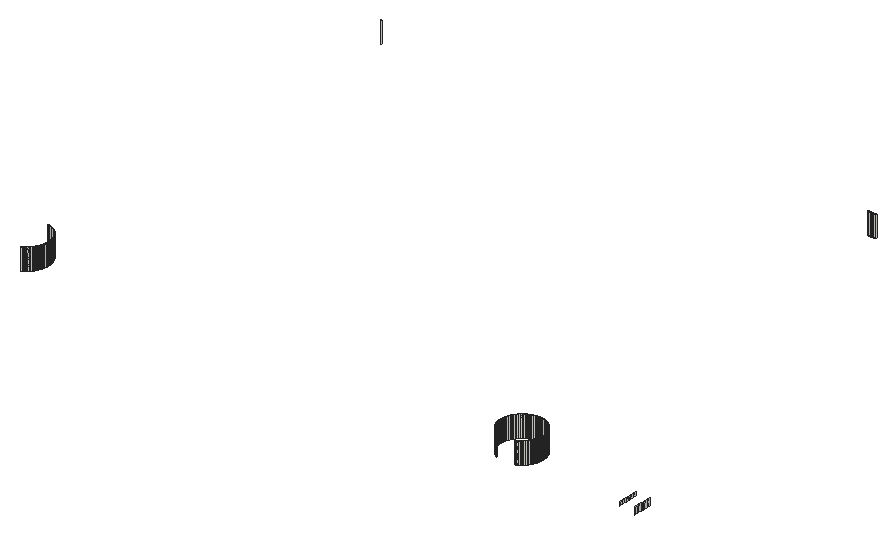
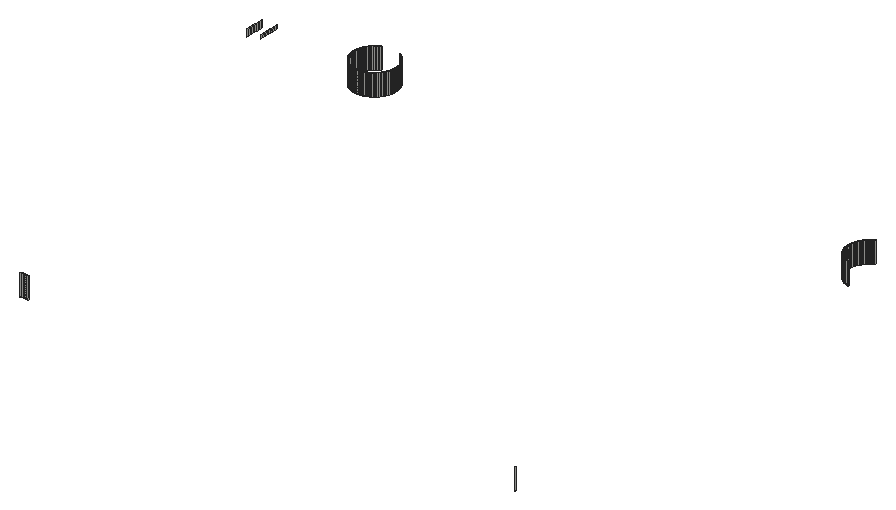
# SketchUp Ruby script. Lengths in inches.
U = 1.inch
M = Sketchup.active_model
def pt(a) = Geom::Point3d.new(a.map { |v| v * U })
def face(e, loops, mat)
  f = e.add_face(loops[0].map { |a| pt(a) })
  loops[1..].each { |l| e.add_face(l.map { |a| pt(a) }).erase! }
  f.material = f.back_material = mat if mat
  f
end
# faces: each face lists its corners as indices into pts; further lists are holes
def faces(e, pts, list, mat = nil) = list.each { |f| face(e, (f[0].is_a?(Array) ? f : [f]).map { |l| l.map { |i| pts[i] } }, mat) }
# xy, xz, yz: faces in a plane at the given z, y or x. An outline is a flat list of corners, or four numbers for a rectangle; further outlines are holes
def ring(l) = l.size == 4 ? [[l[0], l[1]], [l[2], l[1]], [l[2], l[3]], [l[0], l[3]]] : l.each_slice(2).to_a
def flat(e, list, mat, &to3) = list.each { |f| face(e, (f[0].is_a?(Array) ? f : [f]).map { |l| ring(l).map { |u, v| to3.(u, v) } }, mat) }
def xy(e, z, list, mat = nil) = flat(e, list, mat) { |x, y| [x, y, z] }
def xz(e, y, list, mat = nil) = flat(e, list, mat) { |x, z| [x, y, z] }
def yz(e, x, list, mat = nil) = flat(e, list, mat) { |y, z| [x, y, z] }
def lines(e, pts, list) = list.each { |a, b| e.add_line(pt(pts[a]), pt(pts[b])) }
# prism: a flat outline (further loops are holes) pulled along v
def prism(e, loops, v, mat = nil)
  f = face(e, loops, mat); d = Geom::Vector3d.new(v.map { |x| x * U })
  f.pushpull(f.normal.samedirection?(d) ? d.length : -d.length)
end
def box(e, o, s, mat = nil) = prism(e, [[o, [o[0] + s[0], o[1], o[2]], [o[0] + s[0], o[1] + s[1], o[2]], [o[0], o[1] + s[1], o[2]]]], [0, 0, s[2]], mat)
def at(x, y, z, deg = 0) = Geom::Transformation.translation(pt([x, y, z])) * Geom::Transformation.rotation(ORIGIN, Z_AXIS, deg.degrees)
def axes(o, x, y, z) = Geom::Transformation.new([*x, 0, *y, 0, *z, 0, *pt(o).to_a, 1])
def part(name) = M.definitions.add(name)
# library, detail: a bought-in or finely detailed component or shape, given as its bounding box
def library(name, o, s) = part(name).tap { |d| box(d.entities, o, s) }
def detail(e, o, s) = box(e.add_group.entities, o, s)
def put(e, d, t, mat = nil) = e.add_instance(d, t).tap { |i| i.material = mat if mat }
def group(e, t, mat = nil) = e.add_group.tap { |g| g.transformation = t; g.material = mat if mat }.entities
root = M.entities
xz(root,191,[[328.84,108,328.92,111],[328.92,108,329,111],[329,108,329.08,111],[329.08,108,329.16,111]])
xz(root,249.5,[[328.84,108,328.92,111],[328.92,108,329,111],[329,108,329.08,111],[329.08,108,329.16,111]])
yz(root,262.5,[[187.84,108,187.92,111],[187.92,108,188,111],[188,108,188.08,111],[188.08,108,188.16,111]])
yz(root,326,[[187.84,108,187.92,111],[187.92,108,188,111],[188,108,188.08,111],[188.08,108,188.16,111]])
yz(root,332,[[187.84,108,187.92,111],[187.92,108,188,111],[188,108,188.08,111],[188.08,108,188.16,111]])
yz(root,345,[[186.92,108,187.16,108.5],[187.16,108,187.4,108.5],[187.4,108,187.64,108.5],[187.64,108,187.96,108.5]])
yz(root,347,[[186.875,107.5,187.13,108.5],[187.13,107.5,187.39,108.5],[187.39,107.5,187.65,108.5],[187.65,107.5,187.97,108.5]])
p = [[346.94,185.59,107.5],[346.92,185.34,107.5],[346.92,185.34,108.5],[346.94,185.59,108.5],[346.96,185.85,107.5],[346.96,185.85,108.5],
  [346.97,186.1,107.5],[346.97,186.1,108.5],[346.98,186.36,107.5],[346.98,186.36,108.5],[346.99,186.62,107.5],[346.99,186.62,108.5],
  [347,186.875,107.5],[347,186.875,108.5],[344.91,185.25,108],[344.93,185.48,108],[344.93,185.48,108.5],[344.91,185.25,108.5],
  [260.79,185.29,108],[260.72,185.26,108],[260.72,185.26,111],[260.79,185.29,111],[260.86,185.33,108],[260.86,185.33,111],
  [260.93,185.36,108],[260.93,185.36,111],[327.71,185.29,108],[327.64,185.33,108],[327.64,185.33,111],[327.71,185.29,111],
  [327.57,185.36,108],[327.57,185.36,111],[330.29,185.29,108],[330.22,185.26,108],[330.22,185.26,111],[330.29,185.29,111],
  [330.36,185.33,108],[330.36,185.33,111],[330.43,185.36,108],[330.43,185.36,111],[261,185.4,108],[261,185.4,111],
  [261.07,185.44,108],[261.07,185.44,111],[261.13,185.48,108],[261.13,185.48,111],[327.5,185.4,108],[327.43,185.44,108],
  [327.43,185.44,111],[327.5,185.4,111],[327.37,185.48,108],[327.37,185.48,111],[330.5,185.4,108],[330.5,185.4,111],
  [330.57,185.44,108],[330.57,185.44,111],[330.63,185.48,108],[330.63,185.48,111],[261.2,185.53,108],[261.2,185.53,111],
  [261.26,185.57,108],[261.26,185.57,111],[327.3,185.53,108],[327.24,185.57,108],[327.24,185.57,111],[327.3,185.53,111],
  [330.7,185.53,108],[330.7,185.53,111],[330.76,185.57,108],[330.76,185.57,111],[344.95,185.72,108],[344.95,185.72,108.5],
  [261.33,185.62,108],[261.33,185.62,111],[261.39,185.67,108],[261.39,185.67,111],[327.17,185.62,108],[327.11,185.67,108],
  [327.11,185.67,111],[327.17,185.62,111],[330.83,185.62,108],[330.83,185.62,111],[330.89,185.67,108],[330.89,185.67,111],
  [261.45,185.72,108],[261.45,185.72,111],[261.51,185.77,108],[261.51,185.77,111],[327.05,185.72,108],[326.99,185.77,108],
  [326.99,185.77,111],[327.05,185.72,111],[330.95,185.72,108],[330.95,185.72,111],[331.01,185.77,108],[331.01,185.77,111],
  [344.96,185.96,108],[344.96,185.96,108.5],[261.57,185.82,108],[261.57,185.82,111],[261.62,185.88,108],[261.62,185.88,111],
  [326.93,185.82,108],[326.93,185.82,111],[326.88,185.88,108],[326.88,185.88,111],[331.07,185.82,108],[331.07,185.82,111],
  [331.12,185.88,108],[331.12,185.88,111],[261.68,185.93,108],[261.68,185.93,111],[261.73,185.99,108],[261.73,185.99,111],
  [326.82,185.93,108],[326.82,185.93,111],[326.77,185.99,108],[326.77,185.99,111],[331.18,185.93,108],[331.18,185.93,111],
  [331.23,185.99,108],[331.23,185.99,111],[261.78,186.05,108],[261.78,186.05,111],[326.72,186.05,108],[326.72,186.05,111],
  [331.28,186.05,108],[331.28,186.05,111],[344.97,186.2,108],[344.97,186.2,108.5],[261.83,186.11,108],[261.83,186.11,111],
  [261.88,186.17,108],[261.88,186.17,111],[326.67,186.11,108],[326.62,186.17,108],[326.62,186.17,111],[326.67,186.11,111],
  [331.33,186.11,108],[331.33,186.11,111],[331.38,186.17,108],[331.38,186.17,111],[261.93,186.24,108],[261.93,186.24,111],
  [261.97,186.3,108],[261.97,186.3,111],[326.57,186.24,108],[326.53,186.3,108],[326.53,186.3,111],[326.57,186.24,111],
  [331.43,186.24,108],[331.43,186.24,111],[331.47,186.3,108],[331.47,186.3,111],[344.98,186.4375,108],[344.98,186.4375,108.5],
  [262.02,186.37,108],[262.02,186.37,111],[326.48,186.37,108],[326.48,186.37,111],[331.52,186.37,108],[331.52,186.37,111],
  [262.06,186.43,108],[262.06,186.43,111],[262.1,186.5,108],[262.1,186.5,111],[326.44,186.43,108],[326.44,186.43,111],
  [326.4,186.5,108],[326.4,186.5,111],[331.56,186.43,108],[331.56,186.43,111],[331.6,186.5,108],[331.6,186.5,111],
  [344.99,186.68,108],[344.99,186.68,108.5],[262.14,186.57,108],[262.14,186.57,111],[326.36,186.57,108],[326.36,186.57,111],
  [331.64,186.57,108],[331.64,186.57,111],[262.17,186.64,108],[262.17,186.64,111],[262.21,186.71,108],[262.21,186.71,111],
  [326.33,186.64,108],[326.33,186.64,111],[326.29,186.71,108],[326.29,186.71,111],[331.67,186.64,108],[331.67,186.64,111],
  [331.71,186.71,108],[331.71,186.71,111],[262.24,186.78,108],[262.24,186.78,111],[326.26,186.78,108],[326.26,186.78,111],
  [331.74,186.78,108],[331.74,186.78,111],[345,186.92,108],[345,186.92,108.5],[262.27,186.85,108],[262.27,186.85,111],
  [326.23,186.85,108],[326.23,186.85,111],[331.77,186.85,108],[331.77,186.85,111],[262.3,186.92,108],[262.3,186.92,111],
  [262.33,187,108],[262.33,187,111],[326.2,186.92,108],[326.2,186.92,111],[326.17,187,108],[326.17,187,111],
  [331.8,186.92,108],[331.8,186.92,111],[331.83,187,108],[331.83,187,111],[262.35,187.07,108],[262.35,187.07,111],
  [326.15,187.07,108],[326.15,187.07,111],[331.85,187.07,108],[331.85,187.07,111],[262.375,187.15,108],[262.375,187.15,111],
  [262.4,187.22,108],[262.4,187.22,111],[326.125,187.15,108],[326.125,187.15,111],[326.1,187.22,108],[326.1,187.22,111],
  [331.875,187.15,108],[331.875,187.15,111],[331.9,187.22,108],[331.9,187.22,111],[262.42,187.3,108],[262.42,187.3,111],
  [326.08,187.3,108],[326.08,187.3,111],[331.92,187.3,108],[331.92,187.3,111],[262.43,187.375,108],[262.43,187.375,111],
  [326.07,187.375,108],[326.07,187.375,111],[331.93,187.375,108],[331.93,187.375,111],[262.45,187.45,108],[262.45,187.45,111],
  [326.05,187.45,108],[326.05,187.45,111],[331.95,187.45,108],[331.95,187.45,111],[262.46,187.53,108],[262.46,187.53,111],
  [262.47,187.61,108],[262.47,187.61,111],[326.04,187.53,108],[326.04,187.53,111],[326.03,187.61,108],[326.03,187.61,111],
  [331.96,187.53,108],[331.96,187.53,111],[331.97,187.61,108],[331.97,187.61,111],[262.48,187.6875,108],[262.48,187.6875,111],
  [326.02,187.6875,108],[326.02,187.6875,111],[331.98,187.6875,108],[331.98,187.6875,111],[262.49,187.76,108],[262.49,187.76,111],
  [326.01,187.76,108],[326.01,187.76,111],[331.99,187.76,108],[331.99,187.76,111],[262.5,187.84,108],[262.5,187.84,111],
  [326,187.84,108],[326,187.84,111],[332,187.84,108],[332,187.84,111],[262.49,188.24,108],[262.5,188.16,108],
  [262.5,188.16,111],[262.49,188.24,111],[262.48,188.3125,108],[262.48,188.3125,111],[326,188.16,108],[326.01,188.24,108],
  [326.01,188.24,111],[326,188.16,111],[326.02,188.3125,108],[326.02,188.3125,111],[331.99,188.24,108],[332,188.16,108],
  [332,188.16,111],[331.99,188.24,111],[331.98,188.3125,108],[331.98,188.3125,111],[262.47,188.39,108],[262.47,188.39,111],
  [326.03,188.39,108],[326.03,188.39,111],[331.97,188.39,108],[331.97,188.39,111],[262.46,188.47,108],[262.46,188.47,111],
  [326.04,188.47,108],[326.04,188.47,111],[331.96,188.47,108],[331.96,188.47,111],[262.45,188.55,108],[262.45,188.55,111],
  [262.43,188.625,108],[262.43,188.625,111],[326.05,188.55,108],[326.05,188.55,111],[326.07,188.625,108],[326.07,188.625,111],
  [331.95,188.55,108],[331.95,188.55,111],[331.93,188.625,108],[331.93,188.625,111],[262.42,188.7,108],[262.42,188.7,111],
  [326.08,188.7,108],[326.08,188.7,111],[331.92,188.7,108],[331.92,188.7,111],[262.4,188.78,108],[262.4,188.78,111],
  [326.1,188.78,108],[326.1,188.78,111],[331.9,188.78,108],[331.9,188.78,111],[262.375,188.85,108],[262.375,188.85,111],
  [326.125,188.85,108],[326.125,188.85,111],[331.875,188.85,108],[331.875,188.85,111],[262.33,189,108],[262.35,188.93,108],
  [262.35,188.93,111],[262.33,189,111],[326.15,188.93,108],[326.15,188.93,111],[326.17,189,108],[326.17,189,111],
  [331.83,189,108],[331.85,188.93,108],[331.85,188.93,111],[331.83,189,111],[262.3,189.08,108],[262.3,189.08,111],
  [326.2,189.08,108],[326.2,189.08,111],[331.8,189.08,108],[331.8,189.08,111],[262.24,189.22,108],[262.27,189.15,108],
  [262.27,189.15,111],[262.24,189.22,111],[326.23,189.15,108],[326.23,189.15,111],[326.26,189.22,108],[326.26,189.22,111],
  [331.74,189.22,108],[331.77,189.15,108],[331.77,189.15,111],[331.74,189.22,111],[262.21,189.29,108],[262.21,189.29,111],
  [326.29,189.29,108],[326.29,189.29,111],[331.71,189.29,108],[331.71,189.29,111],[262.17,189.36,108],[262.17,189.36,111],
  [326.33,189.36,108],[326.33,189.36,111],[331.67,189.36,108],[331.67,189.36,111],[262.14,189.43,108],[262.14,189.43,111],
  [262.1,189.5,108],[262.1,189.5,111],[326.36,189.43,108],[326.36,189.43,111],[326.4,189.5,108],[326.4,189.5,111],
  [331.64,189.43,108],[331.64,189.43,111],[331.6,189.5,108],[331.6,189.5,111],[262.06,189.57,108],[262.06,189.57,111],
  [326.44,189.57,108],[326.44,189.57,111],[331.56,189.57,108],[331.56,189.57,111],[262.02,189.63,108],[262.02,189.63,111],
  [261.97,189.7,108],[261.97,189.7,111],[326.48,189.63,108],[326.48,189.63,111],[326.53,189.7,108],[326.53,189.7,111],
  [331.52,189.63,108],[331.52,189.63,111],[331.47,189.7,108],[331.47,189.7,111],[261.93,189.76,108],[261.93,189.76,111],
  [326.57,189.76,108],[326.57,189.76,111],[331.43,189.76,108],[331.43,189.76,111],[261.83,189.89,108],[261.88,189.83,108],
  [261.88,189.83,111],[261.83,189.89,111],[326.62,189.83,108],[326.62,189.83,111],[326.67,189.89,108],[326.67,189.89,111],
  [331.33,189.89,108],[331.38,189.83,108],[331.38,189.83,111],[331.33,189.89,111],[261.73,190.01,108],[261.78,189.95,108],
  [261.78,189.95,111],[261.73,190.01,111],[326.72,189.95,108],[326.72,189.95,111],[326.77,190.01,108],[326.77,190.01,111],
  [331.23,190.01,108],[331.28,189.95,108],[331.28,189.95,111],[331.23,190.01,111],[261.68,190.07,108],[261.68,190.07,111],
  [326.82,190.07,108],[326.82,190.07,111],[331.18,190.07,108],[331.18,190.07,111],[261.62,190.12,108],[261.62,190.12,111],
  [261.57,190.18,108],[261.57,190.18,111],[326.88,190.12,108],[326.88,190.12,111],[326.93,190.18,108],[326.93,190.18,111],
  [331.12,190.12,108],[331.12,190.12,111],[331.07,190.18,108],[331.07,190.18,111],[261.45,190.28,108],[261.51,190.23,108],
  [261.51,190.23,111],[261.45,190.28,111],[326.99,190.23,108],[326.99,190.23,111],[327.05,190.28,108],[327.05,190.28,111],
  [330.95,190.28,108],[331.01,190.23,108],[331.01,190.23,111],[330.95,190.28,111],[261.33,190.38,108],[261.39,190.33,108],
  [261.39,190.33,111],[261.33,190.38,111],[327.11,190.33,108],[327.11,190.33,111],[327.17,190.38,108],[327.17,190.38,111],
  [330.83,190.38,108],[330.89,190.33,108],[330.89,190.33,111],[330.83,190.38,111],[261.2,190.47,108],[261.26,190.43,108],
  [261.26,190.43,111],[261.2,190.47,111],[327.24,190.43,108],[327.24,190.43,111],[327.3,190.47,108],[327.3,190.47,111],
  [330.7,190.47,108],[330.76,190.43,108],[330.76,190.43,111],[330.7,190.47,111],[261.13,190.52,108],[261.13,190.52,111],
  [261.07,190.56,108],[261.07,190.56,111],[327.37,190.52,108],[327.37,190.52,111],[327.43,190.56,108],[327.43,190.56,111],
  [330.63,190.52,108],[330.63,190.52,111],[330.57,190.56,108],[330.57,190.56,111],[260.93,190.64,108],[261,190.6,108],
  [261,190.6,111],[260.93,190.64,111],[260.86,190.67,108],[260.86,190.67,111],[327.5,190.6,108],[327.5,190.6,111],
  [327.57,190.64,108],[327.57,190.64,111],[327.64,190.67,108],[327.64,190.67,111],[330.43,190.64,108],[330.5,190.6,108],
  [330.5,190.6,111],[330.43,190.64,111],[330.36,190.67,108],[330.36,190.67,111],[260.65,190.77,108],[260.72,190.74,108],
  [260.72,190.74,111],[260.65,190.77,111],[260.79,190.71,108],[260.79,190.71,111],[327.71,190.71,108],[327.71,190.71,111],
  [327.78,190.74,108],[327.78,190.74,111],[327.85,190.77,108],[327.85,190.77,111],[330.15,190.77,108],[330.22,190.74,108],
  [330.22,190.74,111],[330.15,190.77,111],[330.29,190.71,108],[330.29,190.71,111],[260.43,190.85,108],[260.5,190.83,108],
  [260.5,190.83,111],[260.43,190.85,111],[260.58,190.8,108],[260.58,190.8,111],[327.92,190.8,108],[327.92,190.8,111],
  [328,190.83,108],[328,190.83,111],[328.07,190.85,108],[328.07,190.85,111],[329.93,190.85,108],[330,190.83,108],
  [330,190.83,111],[329.93,190.85,111],[330.08,190.8,108],[330.08,190.8,111],[260.05,190.95,108],[260.125,190.93,108],
  [260.125,190.93,111],[260.05,190.95,111],[259.97,190.96,108],[259.97,190.96,111],[260.2,190.92,108],[260.2,190.92,111],
  [260.28,190.9,108],[260.28,190.9,111],[260.35,190.875,108],[260.35,190.875,111],[328.15,190.875,108],[328.15,190.875,111],
  [328.22,190.9,108],[328.22,190.9,111],[328.3,190.92,108],[328.3,190.92,111],[328.375,190.93,108],[328.375,190.93,111],
  [328.45,190.95,108],[328.45,190.95,111],[328.53,190.96,108],[328.53,190.96,111],[329.55,190.95,108],[329.625,190.93,108],
  [329.625,190.93,111],[329.55,190.95,111],[329.47,190.96,108],[329.47,190.96,111],[329.7,190.92,108],[329.7,190.92,111],
  [329.78,190.9,108],[329.78,190.9,111],[329.85,190.875,108],[329.85,190.875,111],[328.61,190.97,108],[328.61,190.97,111],
  [328.6875,190.98,108],[328.6875,190.98,111],[328.76,190.99,108],[328.76,190.99,111],[328.84,191,108],[328.84,191,111],
  [329.24,190.99,108],[329.3125,190.98,108],[329.3125,190.98,111],[329.24,190.99,111],[329.16,191,108],[329.16,191,111],
  [329.39,190.97,108],[329.39,190.97,111],[259.97,249.54,108],[259.89,249.53,108],[259.89,249.53,111],[259.97,249.54,111],
  [260.05,249.55,108],[260.05,249.55,111],[328.61,249.53,108],[328.53,249.54,108],[328.53,249.54,111],[328.61,249.53,111],
  [328.45,249.55,108],[328.45,249.55,111],[328.6875,249.52,108],[328.6875,249.52,111],[328.76,249.51,108],[328.76,249.51,111],
  [328.84,249.5,108],[328.84,249.5,111],[329.24,249.51,108],[329.16,249.5,108],[329.16,249.5,111],[329.24,249.51,111],
  [329.3125,249.52,108],[329.3125,249.52,111],[329.39,249.53,108],[329.39,249.53,111],[329.47,249.54,108],[329.47,249.54,111],
  [329.55,249.55,108],[329.55,249.55,111],[328.375,249.57,108],[328.375,249.57,111]]
faces(root,p,[[0,1,2,3],[4,0,3,5],[6,4,5,7],[8,6,7,9],[10,8,9,11],[12,10,11,13],[14,15,16,17],[18,19,20,21],
  [22,18,21,23],[24,22,23,25],[26,27,28,29],[27,30,31,28],[32,33,34,35],[36,32,35,37],[38,36,37,39],[40,24,25,41],
  [42,40,41,43],[44,42,43,45],[46,47,48,49],[47,50,51,48],[30,46,49,31],[52,38,39,53],[54,52,53,55],[56,54,55,57],
  [58,44,45,59],[60,58,59,61],[62,63,64,65],[50,62,65,51],[66,56,57,67],[68,66,67,69],[15,70,71,16],[72,60,61,73],
  [74,72,73,75],[76,77,78,79],[63,76,79,64],[80,68,69,81],[82,80,81,83],[84,74,75,85],[86,84,85,87],[88,89,90,91],
  [77,88,91,78],[92,82,83,93],[94,92,93,95],[70,96,97,71],[98,86,87,99],[100,98,99,101],[89,102,103,90],[102,104,105,103],
  [106,94,95,107],[108,106,107,109],[110,100,101,111],[112,110,111,113],[104,114,115,105],[114,116,117,115],[118,108,109,119],[120,118,119,121],
  [122,112,113,123],[116,124,125,117],[126,120,121,127],[96,128,129,97],[130,122,123,131],[132,130,131,133],[134,135,136,137],[124,134,137,125],
  [138,126,127,139],[140,138,139,141],[142,132,133,143],[144,142,143,145],[146,147,148,149],[135,146,149,136],[150,140,141,151],[152,150,151,153],
  [128,154,155,129],[156,144,145,157],[147,158,159,148],[160,152,153,161],[162,156,157,163],[164,162,163,165],[158,166,167,159],[166,168,169,167],
  [170,160,161,171],[172,170,171,173],[154,174,175,155],[176,164,165,177],[168,178,179,169],[180,172,173,181],[182,176,177,183],[184,182,183,185],
  [178,186,187,179],[186,188,189,187],[190,180,181,191],[192,190,191,193],[194,184,185,195],[188,196,197,189],[198,192,193,199],[174,200,201,175],
  [202,194,195,203],[196,204,205,197],[206,198,199,207],[208,202,203,209],[210,208,209,211],[204,212,213,205],[212,214,215,213],[216,206,207,217],
  [218,216,217,219],[220,210,211,221],[214,222,223,215],[224,218,219,225],[226,220,221,227],[228,226,227,229],[222,230,231,223],[230,232,233,231],
  [234,224,225,235],[236,234,235,237],[238,228,229,239],[232,240,241,233],[242,236,237,243],[244,238,239,245],[240,246,247,241],[248,242,243,249],
  [250,244,245,251],[246,252,253,247],[254,248,249,255],[256,250,251,257],[258,256,257,259],[252,260,261,253],[260,262,263,261],[264,254,255,265],
  [266,264,265,267],[268,258,259,269],[262,270,271,263],[272,266,267,273],[274,268,269,275],[270,276,277,271],[278,272,273,279],[280,274,275,281],
  [276,282,283,277],[284,278,279,285],[286,287,288,289],[290,286,289,291],[292,293,294,295],[293,296,297,294],[298,299,300,301],[302,298,301,303],
  [304,290,291,305],[296,306,307,297],[308,302,303,309],[310,304,305,311],[306,312,313,307],[314,308,309,315],[316,310,311,317],[318,316,317,319],
  [312,320,321,313],[320,322,323,321],[324,314,315,325],[326,324,325,327],[328,318,319,329],[322,330,331,323],[332,326,327,333],[334,328,329,335],
  [330,336,337,331],[338,332,333,339],[340,334,335,341],[336,342,343,337],[344,338,339,345],[346,347,348,349],[347,340,341,348],[342,350,351,343],
  [350,352,353,351],[354,355,356,357],[355,344,345,356],[358,346,349,359],[352,360,361,353],[362,354,357,363],[364,365,366,367],[365,358,359,366],
  [360,368,369,361],[368,370,371,369],[372,373,374,375],[373,362,363,374],[376,364,367,377],[370,378,379,371],[380,372,375,381],[382,376,377,383],
  [378,384,385,379],[386,380,381,387],[388,382,383,389],[390,388,389,391],[384,392,393,385],[392,394,395,393],[396,386,387,397],[398,396,397,399],
  [400,390,391,401],[394,402,403,395],[404,398,399,405],[406,400,401,407],[408,406,407,409],[402,410,411,403],[410,412,413,411],[414,404,405,415],
  [416,414,415,417],[418,408,409,419],[412,420,421,413],[422,416,417,423],[424,425,426,427],[425,418,419,426],[420,428,429,421],[428,430,431,429],
  [432,433,434,435],[433,422,423,434],[436,437,438,439],[437,424,427,438],[430,440,441,431],[440,442,443,441],[444,445,446,447],[445,432,435,446],
  [448,436,439,449],[442,450,451,443],[452,444,447,453],[454,448,449,455],[456,454,455,457],[450,458,459,451],[458,460,461,459],[462,452,453,463],
  [464,462,463,465],[466,467,468,469],[467,456,457,468],[460,470,471,461],[470,472,473,471],[474,475,476,477],[475,464,465,476],[478,479,480,481],
  [479,466,469,480],[472,482,483,473],[482,484,485,483],[486,487,488,489],[487,474,477,488],[490,491,492,493],[491,478,481,492],[484,494,495,485],
  [494,496,497,495],[498,499,500,501],[499,486,489,500],[502,490,493,503],[504,502,503,505],[496,506,507,497],[506,508,509,507],[510,498,501,511],
  [512,510,511,513],[514,515,516,517],[518,514,517,519],[515,504,505,516],[508,520,521,509],[520,522,523,521],[522,524,525,523],[526,527,528,529],
  [530,526,529,531],[527,512,513,528],[532,533,534,535],[533,536,537,534],[536,518,519,537],[524,538,539,525],[538,540,541,539],[540,542,543,541],
  [544,545,546,547],[545,548,549,546],[548,530,531,549],[550,551,552,553],[551,554,555,552],[554,532,535,555],[542,556,557,543],[556,558,559,557],
  [558,560,561,559],[562,563,564,565],[563,566,567,564],[566,544,547,567],[568,569,570,571],[572,568,571,573],[569,574,575,570],[574,576,577,575],
  [576,578,579,577],[578,550,553,579],[560,580,581,561],[580,582,583,581],[582,584,585,583],[584,586,587,585],[586,588,589,587],[588,590,591,589],
  [592,593,594,595],[596,592,595,597],[593,598,599,594],[598,600,601,599],[600,602,603,601],[602,562,565,603],[590,604,605,591],[604,606,607,605],
  [606,608,609,607],[608,610,611,609],[612,613,614,615],[616,612,615,617],[613,618,619,614],[618,596,597,619],[620,621,622,623],[624,620,623,625],
  [626,627,628,629],[627,630,631,628],[632,626,629,633],[634,632,633,635],[636,634,635,637],[638,639,640,641],[642,638,641,643],[644,642,643,645],
  [646,644,645,647],[648,646,647,649],[630,650,651,631]])
